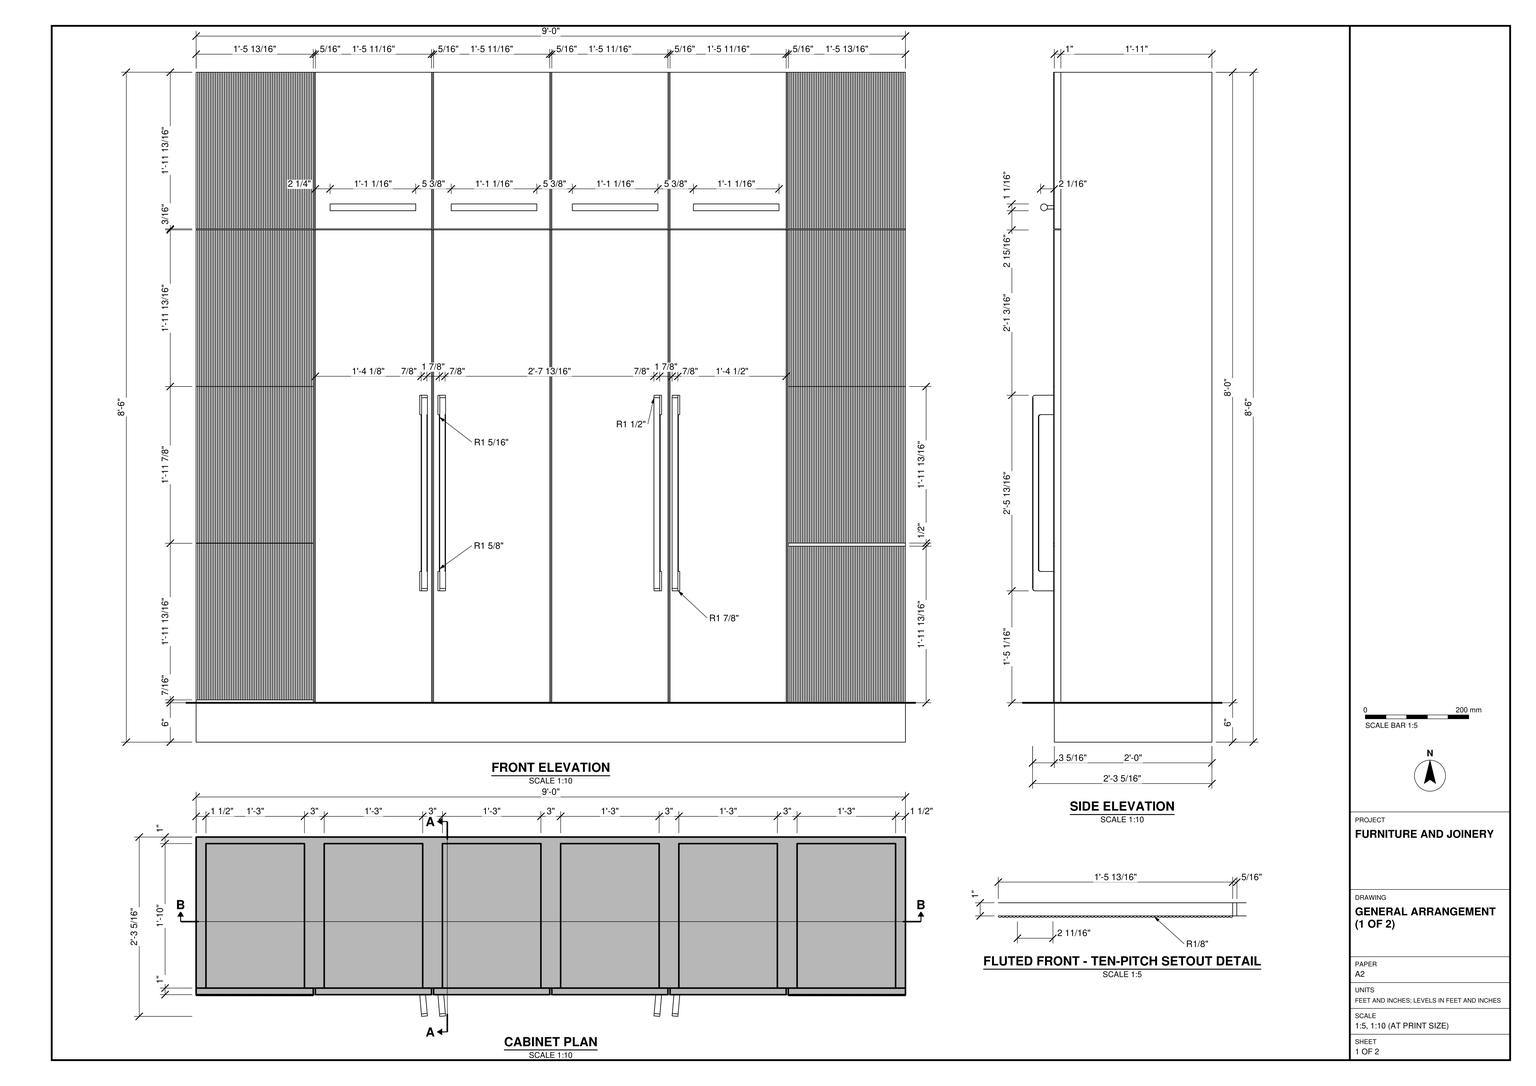
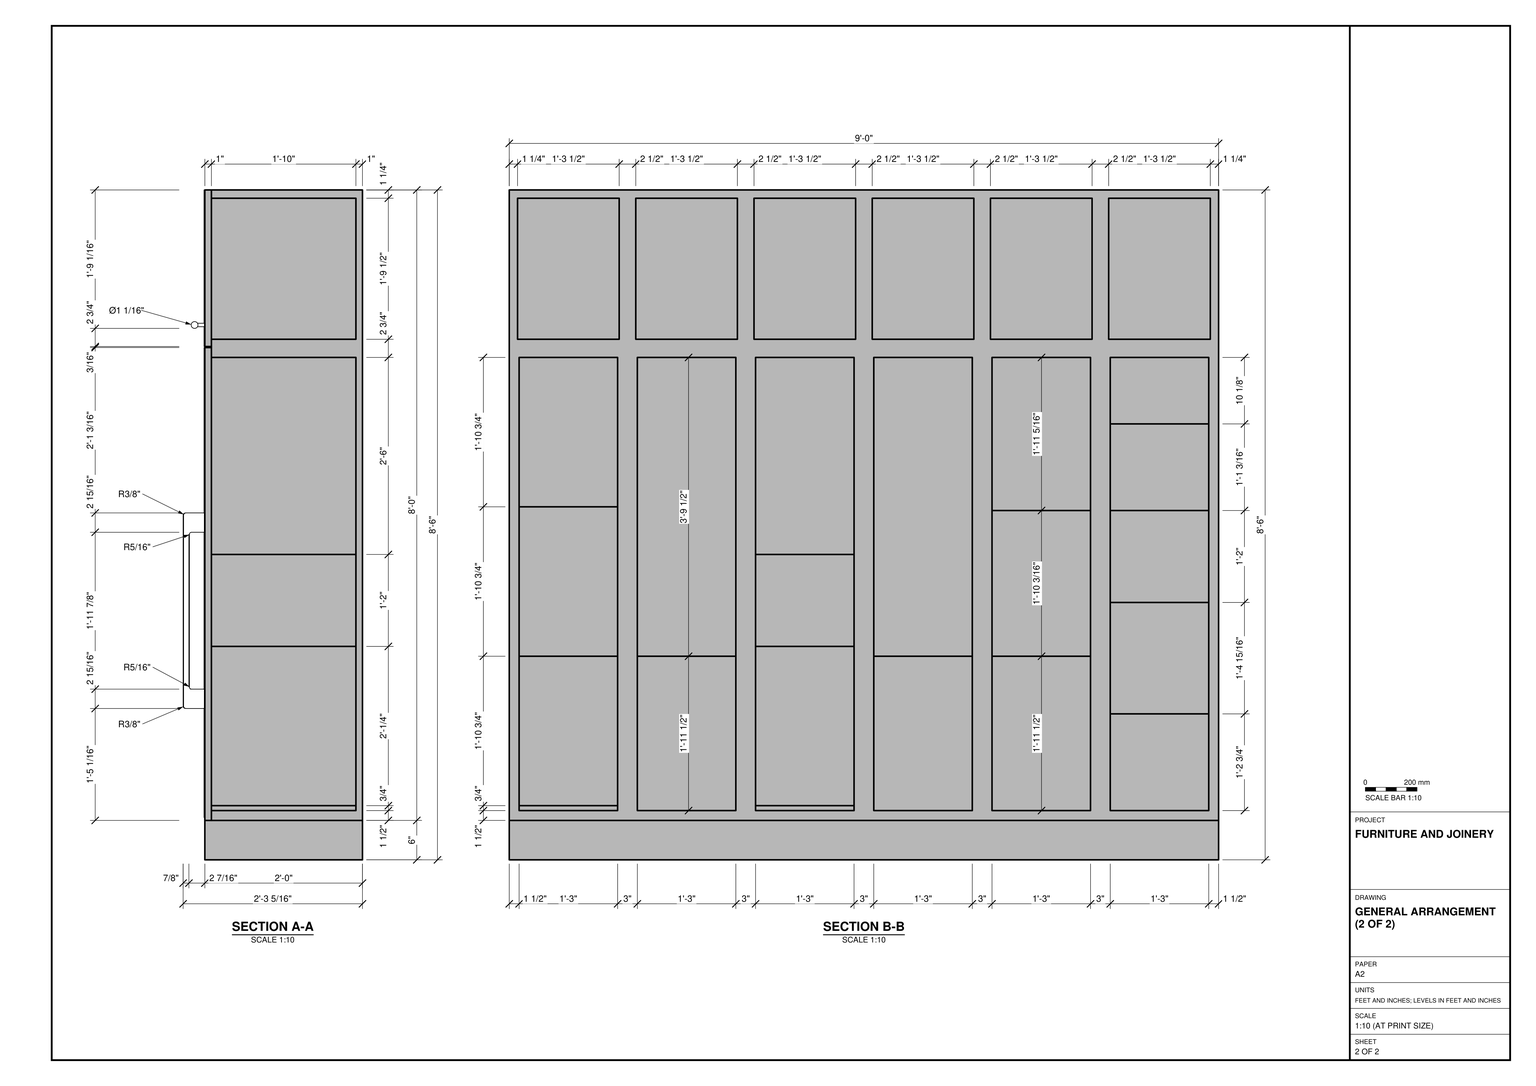
Build the wardrobe in SketchUp from task_files/diagram_01.pdf. Work in feet and inches, with the underside of the plinth at the floor level of ±0'-0". Set the width along the X axis to 9'-0", the overall depth along the Y axis to 2'-3 5/16", and the height to 8'-6". The overall depth includes the projecting pulls; the depth from the back to the closed fronts is 2'-0".

Build the full-width 6" plinth and the cabinet above it. Use the plan and sections to set out the sides, back, top, base, dividers and shelves at the thicknesses shown. Form a row of separate upper compartments and follow section B-B for the shelf heights in each bay below. Do not carry a shelf across a bay that the section shows as open at that height.

Model the fronts closed, keeping the narrow gaps shown in the front elevation. Give the stacked fronts at both ends a vertical fluted profile using the enlarged setout detail. Across the middle, fit short upper doors with horizontal pulls above tall doors with paired vertical pulls. Use the side view to set the pulls clear of the door faces. Keep the cabinet parts, fronts and hardware separately editable as groups or components, and use components for repeated parts. Decor and loose items, if included, may be any suitable library components. Save one SketchUp model as output_files/six_bay_wardrobe_with_fluted_end_fronts.skp.

# SketchUp Ruby script. Lengths in inches.
U = 1.inch
M = Sketchup.active_model
def pt(a) = Geom::Point3d.new(a.map { |v| v * U })
def face(e, loops, mat)
  f = e.add_face(loops[0].map { |a| pt(a) })
  loops[1..].each { |l| e.add_face(l.map { |a| pt(a) }).erase! }
  f.material = f.back_material = mat if mat
  f
end
# faces: each face lists its corners as indices into pts; further lists are holes
def faces(e, pts, list, mat = nil) = list.each { |f| face(e, (f[0].is_a?(Array) ? f : [f]).map { |l| l.map { |i| pts[i] } }, mat) }
# xy, xz, yz: faces in a plane at the given z, y or x. An outline is a flat list of corners, or four numbers for a rectangle; further outlines are holes
def ring(l) = l.size == 4 ? [[l[0], l[1]], [l[2], l[1]], [l[2], l[3]], [l[0], l[3]]] : l.each_slice(2).to_a
def flat(e, list, mat, &to3) = list.each { |f| face(e, (f[0].is_a?(Array) ? f : [f]).map { |l| ring(l).map { |u, v| to3.(u, v) } }, mat) }
def xy(e, z, list, mat = nil) = flat(e, list, mat) { |x, y| [x, y, z] }
def xz(e, y, list, mat = nil) = flat(e, list, mat) { |x, z| [x, y, z] }
def yz(e, x, list, mat = nil) = flat(e, list, mat) { |y, z| [x, y, z] }
def lines(e, pts, list) = list.each { |a, b| e.add_line(pt(pts[a]), pt(pts[b])) }
# prism: a flat outline (further loops are holes) pulled along v
def prism(e, loops, v, mat = nil)
  f = face(e, loops, mat); d = Geom::Vector3d.new(v.map { |x| x * U })
  f.pushpull(f.normal.samedirection?(d) ? d.length : -d.length)
end
def box(e, o, s, mat = nil) = prism(e, [[o, [o[0] + s[0], o[1], o[2]], [o[0] + s[0], o[1] + s[1], o[2]], [o[0], o[1] + s[1], o[2]]]], [0, 0, s[2]], mat)
def at(x, y, z, deg = 0) = Geom::Transformation.translation(pt([x, y, z])) * Geom::Transformation.rotation(ORIGIN, Z_AXIS, deg.degrees)
def axes(o, x, y, z) = Geom::Transformation.new([*x, 0, *y, 0, *z, 0, *pt(o).to_a, 1])
def part(name) = M.definitions.add(name)
# library, detail: a bought-in or finely detailed component or shape, given as its bounding box
def library(name, o, s) = part(name).tap { |d| box(d.entities, o, s) }
def detail(e, o, s) = box(e.add_group.entities, o, s)
def put(e, d, t, mat = nil) = e.add_instance(d, t).tap { |i| i.material = mat if mat }
def group(e, t, mat = nil) = e.add_group.tap { |g| g.transformation = t; g.material = mat if mat }.entities
root = M.entities
M.materials.add("Asian Paints_Archi Concrete Slab Effect_Rocky Terrain").color = [186, 177, 158]
M.materials.add("Asian Paints_Stellato_White Silver").color = [203, 204, 196]
M.materials.add("[0014_DarkSalmon]").color = [233, 150, 122]
M.materials.add("[Color B01]").color = [255, 216, 204]
M.materials.add("[Color C01]").color = [255, 229, 204]
M.materials.add("[Color M09]").color = [0, 0, 0]
M.materials.add("[Granite Dark Gray]").color = [69, 68, 68]
M.materials.add("[Wood Floor Parquet]").color = [142, 87, 38]
c1 = part("tubular wardrobe handle")
g1 = group(c1.entities,at(0,0,0),"[Color B01]")
xy(g1,0,[[0.197,0,0.591,0.984],[0.197,8.858,0.591,9.843]])
xy(g1,0.844,[[0.197,0.984,0.591,8.858]])
xz(g1,0,[[0.197,0,0.591,0,0.591,0.844,0.536,0.814,0.436,0.79,0.333,0.792,0.235,0.821,0.197,0.844],[0.436,0.79,0.536,0.814,0.591,0.844,0.626,0.863,0.7,0.934,0.754,1.022,0.783,1.121,0.784,1.181,0.785,1.223,0.761,1.323,0.712,1.413,0.641,1.488,0.553,1.541,0.454,1.57,0.351,1.573,0.252,1.548,0.161,1.499,0.087,1.428,0.034,1.34,0.005,1.242,0.003,1.181,0.002,1.139,0.027,1.039,0.076,0.949,0.147,0.874,0.197,0.844,0.235,0.821,0.333,0.792]])
xz(g1,0.984,[[0.197,0,0.591,0.844]])
xz(g1,8.858,[[0.197,0,0.591,0.844]])
xz(g1,9.843,[[0.197,0,0.197,0.844,0.235,0.821,0.333,0.792,0.436,0.79,0.536,0.814,0.591,0.844,0.591,0],[0.436,0.79,0.333,0.792,0.235,0.821,0.197,0.844,0.147,0.874,0.076,0.949,0.027,1.039,0.002,1.139,0.005,1.242,0.034,1.34,0.087,1.428,0.161,1.499,0.252,1.548,0.351,1.573,0.454,1.57,0.553,1.541,0.641,1.488,0.712,1.413,0.761,1.323,0.785,1.223,0.783,1.121,0.754,1.022,0.7,0.934,0.626,0.863,0.591,0.844,0.536,0.814]])
yz(g1,0.197,[[0,0,0.984,0.844],[8.858,0,9.843,0.844]])
yz(g1,0.591,[[0,0,0.984,0.844],[8.858,0,9.843,0.844]])
p = [[0.147,9.843,0.874],[0.197,9.843,0.844],[0.197,8.858,0.844],[0.197,0.984,0.844],[0.197,0,0.844],[0.147,0,0.874],
  [0.235,0,0.821],[0.235,9.843,0.821],[0.333,0,0.792],[0.333,9.843,0.792],[0.436,0,0.79],[0.436,9.843,0.79],
  [0.536,0,0.814],[0.536,9.843,0.814],[0.591,0,0.844],[0.591,9.843,0.844],[0.591,8.858,0.844],[0.591,0.984,0.844],
  [0.626,0,0.863],[0.626,9.843,0.863],[0.076,0,0.949],[0.027,0,1.039],[0.027,9.843,1.039],[0.076,9.843,0.949],
  [0.7,0,0.934],[0.7,9.843,0.934],[0.754,0,1.022],[0.754,9.843,1.022],[0.002,0,1.139],[0.002,9.843,1.139],
  [0.783,0,1.121],[0.783,9.843,1.121],[0.003,0,1.181],[0.005,0,1.242],[0.005,9.843,1.242],[0.785,0,1.223],
  [0.784,0,1.181],[0.785,9.843,1.223],[0.034,0,1.34],[0.034,9.843,1.34],[0.761,0,1.323],[0.761,9.843,1.323],
  [0.087,0,1.428],[0.087,9.843,1.428],[0.712,0,1.413],[0.712,9.843,1.413],[0.161,0,1.499],[0.161,9.843,1.499],
  [0.641,0,1.488],[0.641,9.843,1.488],[0.252,0,1.548],[0.252,9.843,1.548],[0.351,0,1.573],[0.351,9.843,1.573],
  [0.454,0,1.57],[0.553,0,1.541],[0.553,9.843,1.541],[0.454,9.843,1.57],[0.787,0,1.181],[0,0,1.181]]
faces(g1,p,[[0,1,2,3,4,5],[6,4,3,2,1,7],[8,6,7,9],[10,8,9,11],[12,10,11,13],[14,12,13,15,16,17],[18,14,17,16,15,19],[20,21,22,23],
  [5,20,23,0],[24,18,19,25],[26,24,25,27],[21,28,29,22],[30,26,27,31],[28,32,33,34,29],[35,36,30,31,37],[33,38,39,34],
  [40,35,37,41],[38,42,43,39],[44,40,41,45],[42,46,47,43],[48,44,45,49],[46,50,51,47],[50,52,53,51],[54,55,56,57],
  [55,48,49,56],[52,54,57,53]])
lines(g1,p,[[58,36],[59,32]])
c2 = part("Modern+Drawer+Handle+10+inch+01")
g2 = group(c2.entities,at(0,0,0),"[Color C01]")
yz(g2,0,[[-1,-0.09,-1.03,0.21,-1.01,0.21,-0.99,-0.09],[-0.99,-0.09,-1.01,0.21,-1,0.21,-0.97,-0.08],[-0.97,-0.08,-1,0.21,-0.03,0.3,0,0]])
yz(g2,1,[[-0.72,-0.0625,-0.71,-0.0625,-0.73,0.24,-0.75,0.24],[-0.71,-0.0625,-0.6875,-0.06,-0.72,0.24,-0.73,0.24],[-0.6875,-0.06,-0.67,-0.06,-0.7,0.24,-0.72,0.24],[-0.67,-0.06,0,0,-0.03,0.3,-0.7,0.24]])
yz(g2,9.1,[[-0.72,-0.0625,-0.75,0.24,-0.73,0.24,-0.71,-0.0625],[-0.71,-0.0625,-0.73,0.24,-0.72,0.24,-0.6875,-0.06],[-0.6875,-0.06,-0.72,0.24,-0.7,0.24,-0.67,-0.06],[-0.67,-0.06,-0.7,0.24,-0.03,0.3,0,0]])
yz(g2,10.1,[[-1,-0.09,-0.99,-0.09,-1.01,0.21,-1.03,0.21],[-0.99,-0.09,-0.97,-0.08,-1,0.21,-1.01,0.21],[-0.97,-0.08,0,0,-0.03,0.3,-1,0.21]])
p = [[0.04,-1.06,-0.09],[0.05,-1.07,-0.09],[0.05,-1.1,0.21],[0.04,-1.09,0.21],[0.02,-1.03,-0.09],[0.03,-1.05,-0.09],
  [0.03,-1.07,0.21],[0.02,-1.06,0.21],[0.0625,-1.08,-0.09],[0.0625,-1.11,0.2],[9.97,-1.1,-0.1],[0.125,-1.1,-0.1],
  [0.11,-1.09,-0.1],[0.09,-1.09,-0.1],[0.08,-1.09,-0.1],[0.01,-1.02,-0.09],[0,-1,-0.09],[0,-0.99,-0.09],
  [0,-0.97,-0.08],[0,0,0],[1,0,0],[1,-0.67,-0.06],[1,-0.6875,-0.06],[1,-0.71,-0.0625],
  [1,-0.72,-0.0625],[1.01,-0.74,-0.06],[1.02,-0.75,-0.07],[1.03,-0.77,-0.07],[1.04,-0.78,-0.07],[1.06,-0.79,-0.07],
  [1.07,-0.79,-0.07],[1.09,-0.8,-0.07],[1.11,-0.8,-0.07],[1.125,-0.8,-0.07],[8.97,-0.8,-0.07],[8.99,-0.8,-0.07],
  [9.01,-0.8,-0.07],[9.03,-0.79,-0.07],[9.04,-0.79,-0.07],[9.06,-0.78,-0.07],[9.07,-0.77,-0.07],[9.08,-0.75,-0.07],
  [9.09,-0.74,-0.06],[9.1,-0.72,-0.0625],[9.1,-0.71,-0.0625],[9.1,-0.6875,-0.06],[9.1,-0.67,-0.06],[9.1,0,0],
  [10.1,0,0],[10.1,-0.97,-0.08],[10.1,-0.99,-0.09],[10.1,-1,-0.09],[10.09,-1.02,-0.09],[10.08,-1.03,-0.09],
  [10.07,-1.05,-0.09],[10.0625,-1.06,-0.09],[10.05,-1.07,-0.09],[10.04,-1.08,-0.09],[10.02,-1.09,-0.1],[10.01,-1.09,-0.1],
  [9.99,-1.09,-0.1],[0.01,-1.05,0.21],[9.97,-1.12,0.2],[0.125,-1.12,0.2],[0.11,-1.12,0.2],[0.09,-1.12,0.2],
  [0.08,-1.11,0.2],[10.01,-1.12,0.2],[9.99,-1.12,0.2],[10.04,-1.11,0.2],[10.02,-1.11,0.2],[10.05,-1.1,0.21],
  [10.08,-1.06,0.21],[10.07,-1.07,0.21],[10.0625,-1.09,0.21],[10.09,-1.05,0.21],[0,-1.03,0.21],[10.1,-1.03,0.21],
  [1.01,-0.76,0.23],[1.02,-0.78,0.23],[1.03,-0.79,0.23],[1.04,-0.8,0.23],[1.06,-0.8125,0.23],[1,-0.75,0.24],
  [1.07,-0.82,0.23],[1.09,-0.82,0.23],[1.11,-0.82,0.23],[1.125,-0.82,0.23],[8.97,-0.82,0.23],[8.99,-0.82,0.23],
  [9.01,-0.82,0.23],[9.03,-0.82,0.23],[9.04,-0.8125,0.23],[9.06,-0.8,0.23],[9.07,-0.79,0.23],[9.08,-0.78,0.23],
  [9.09,-0.76,0.23],[9.1,-0.75,0.24],[0,-0.03,0.3],[1,-0.03,0.3],[9.1,-0.03,0.3],[10.1,-0.03,0.3],
  [9.1,-0.7,0.24],[9.1,-0.72,0.24],[9.1,-0.73,0.24],[1,-0.73,0.24],[1,-0.72,0.24],[1,-0.7,0.24],
  [0,-1,0.21],[0,-1.01,0.21],[10.1,-1.01,0.21],[10.1,-1,0.21]]
faces(g2,p,[[0,1,2,3],[4,5,6,7],[1,8,9,2],[5,0,3,6],[10,11,12,13,14,8,1,0,5,4,15,16,17,18,19,20,21,22,23,24,25,26,27,28,29,30,31,32,33,34,35,36,37,38,39,40,41,42,43,44,45,46,47,48,49,50,51,52,53,54,55,56,57,58,59,60],[15,4,7,61],[13,12,64,65],[8,14,66,9],
  [12,11,63,64],[14,13,65,66],[60,59,67,68],[58,57,69,70],[57,56,71,69],[59,58,70,67],[10,60,68,62],[54,53,72,73],
  [56,55,74,71],[55,54,73,74],[53,52,75,72],[16,15,61,76],[52,51,77,75],[26,25,78,79],[28,27,80,81],[29,28,81,82],
  [25,24,83,78],[27,26,79,80],[31,30,84,85],[33,32,86,87],[32,31,85,86],[34,33,87,88],[30,29,82,84],[35,34,88,89],
  [37,36,90,91],[36,35,89,90],[39,38,92,93],[38,37,91,92],[41,40,94,95],[40,39,93,94],[43,42,96,97],[42,41,95,96],
  [98,99,20,19],[47,100,101,48],[101,100,102,103,104,97,96,95,94,93,92,91,90,89,88,87,86,85,84,82,81,80,79,78,83,105,106,107,99,98,108,109,76,61,7,6,3,2,9,66,65,64,63,62,68,67,70,69,71,74,73,72,75,77,110,111]])
faces(g2,p,[[10,62,63,11]],"[Color C01]")
c3 = part("Fluting strip")
xy(c3.entities,-23.84,[[0.09,0,0.0625,0.02,0.04,0.04,0.02,0.0625,0,0.09,0,0.125,0.25,0.125,0.25,0.09,0.23,0.0625,0.21,0.04,0.1875,0.02,0.16,0]])
xy(c3.entities,0,[[0.09,0,0.16,0,0.1875,0.02,0.21,0.04,0.23,0.0625,0.25,0.09,0.25,0.125,0,0.125,0,0.09,0.02,0.0625,0.04,0.04,0.0625,0.02]])
xz(c3.entities,0,[[0.09,-23.84,0.125,0],[0.125,-23.84,0.16,0]],"[0014_DarkSalmon]")
xz(c3.entities,0.125,[[0,-23.84,0.25,0]])
yz(c3.entities,0,[[0.09,-23.84,0.125,0]],"[0014_DarkSalmon]")
yz(c3.entities,0.25,[[0.09,-23.84,0.125,0]],"[0014_DarkSalmon]")
p = [[0.04,0.04,0],[0.02,0.0625,0],[0.02,0.0625,-23.84],[0.04,0.04,-23.84],[0.0625,0.02,0],[0.0625,0.02,-23.84],
  [0.09,0,0],[0.09,0,-23.84],[0.1875,0.02,0],[0.16,0,0],[0.16,0,-23.84],[0.1875,0.02,-23.84],
  [0.21,0.04,0],[0.21,0.04,-23.84],[0.23,0.0625,0],[0.23,0.0625,-23.84],[0,0.09,0],[0,0.09,-23.84],
  [0.25,0.09,0],[0.25,0.09,-23.84]]
faces(c3.entities,p,[[0,1,2,3],[4,0,3,5],[6,4,5,7],[8,9,10,11],[12,8,11,13],[14,12,13,15],[1,16,17,2],[18,14,15,19]],"[0014_DarkSalmon]")
c4 = part("Fluted front panel")
put(c4.entities,c3,at(11.91,0,23.84))
put(c4.entities,c3,at(12.18,0,23.84))
put(c4.entities,c3,at(7.85,0,23.84))
put(c4.entities,c3,at(8.39,0,23.84))
put(c4.entities,c3,at(12.72,0,23.84))
put(c4.entities,c3,at(4.87,0,23.84))
put(c4.entities,c3,at(6.77,0,23.84))
put(c4.entities,c3,at(3.79,0,23.84))
put(c4.entities,c3,at(1.89,0,23.84))
put(c4.entities,c3,at(7.31,0,23.84))
put(c4.entities,c3,at(2.4375,0,23.84))
put(c4.entities,c3,at(3.25,0,23.84))
put(c4.entities,c3,at(6.5,0,23.84))
put(c4.entities,c3,at(0.27,0,23.84))
put(c4.entities,c3,at(0.54,0,23.84))
put(c4.entities,c3,at(3.52,0,23.84))
put(c4.entities,c3,at(10.28,0,23.84))
put(c4.entities,c3,at(9.74,0,23.84))
put(c4.entities,c3,at(8.66,0,23.84))
put(c4.entities,c3,at(10.83,0,23.84))
put(c4.entities,c3,at(10.01,0,23.84))
put(c4.entities,c3,at(0,0,23.84))
put(c4.entities,c3,at(14.34,0,23.84))
put(c4.entities,c3,at(7.58,0,23.84))
put(c4.entities,c3,at(8.93,0,23.84))
put(c4.entities,c3,at(11.64,0,23.84))
put(c4.entities,c3,at(17.05,0,23.84))
put(c4.entities,c3,at(16.51,0,23.84))
put(c4.entities,c3,at(17.59,0,23.84))
put(c4.entities,c3,at(16.78,0,23.84))
put(c4.entities,c3,at(17.32,0,23.84))
put(c4.entities,c3,at(15.7,0,23.84))
put(c4.entities,c3,at(14.62,0,23.84))
put(c4.entities,c3,at(13.26,0,23.84))
put(c4.entities,c3,at(14.07,0,23.84))
put(c4.entities,c3,at(8.12,0,23.84))
put(c4.entities,c3,at(10.56,0,23.84))
put(c4.entities,c3,at(11.1,0,23.84))
put(c4.entities,c3,at(9.2,0,23.84))
put(c4.entities,c3,at(12.99,0,23.84))
put(c4.entities,c3,at(5.95,0,23.84))
put(c4.entities,c3,at(5.68,0,23.84))
put(c4.entities,c3,at(1.08,0,23.84))
put(c4.entities,c3,at(5.41,0,23.84))
put(c4.entities,c3,at(4.06,0,23.84))
put(c4.entities,c3,at(1.35,0,23.84))
put(c4.entities,c3,at(1.625,0,23.84))
put(c4.entities,c3,at(2.71,0,23.84))
put(c4.entities,c3,at(4.6,0,23.84))
put(c4.entities,c3,at(2.17,0,23.84))
put(c4.entities,c3,at(0.8125,0,23.84))
put(c4.entities,c3,at(4.33,0,23.84))
put(c4.entities,c3,at(5.14,0,23.84))
put(c4.entities,c3,at(9.47,0,23.84))
put(c4.entities,c3,at(13.8,0,23.84))
put(c4.entities,c3,at(11.37,0,23.84))
put(c4.entities,c3,at(13.53,0,23.84))
put(c4.entities,c3,at(12.45,0,23.84))
put(c4.entities,c3,at(15.97,0,23.84))
put(c4.entities,c3,at(16.24,0,23.84))
put(c4.entities,c3,at(14.89,0,23.84))
put(c4.entities,c3,at(15.16,0,23.84))
put(c4.entities,c3,at(15.43,0,23.84))
put(c4.entities,c3,at(7.04,0,23.84))
put(c4.entities,c3,at(2.98,0,23.84))
put(c4.entities,c3,at(6.23,0,23.84))
c5 = part("Group\#7")
xy(c5.entities,0.75,[[0,0,15,22]])
xz(c5.entities,0,[[0,0,15,0.75]])
p = [[18,4.31,23.375],[18.31,4.31,23.375]]
lines(root,p,[[0,1]])
put(root,c1,axes([33.4375,3.31,80.92],[0,0,1.32422],[-1.32422,0,0],[0,-1.32422,0]))
put(root,c2,axes([34.93,3.31,23.04],[0,0,2.94868],[0,2.94868,0],[-2.94868,0,0]))
put(root,c2,axes([37.7,3.31,23.04],[0,0,2.94868],[0,2.94868,0],[-2.94868,0,0]))
put(root,c2,axes([72.75,3.31,23.04],[0,0,2.94868],[0,2.94868,0],[2.94868,0,0]))
put(root,c2,axes([69.99,3.31,23.04],[0,0,2.94868],[0,2.94868,0],[2.94868,0,0]))
put(root,c1,axes([51.875,3.31,80.92],[0,0,1.32422],[-1.32422,0,0],[0,-1.32422,0]))
put(root,c1,axes([70.3125,3.31,80.92],[0,0,1.32422],[-1.32422,0,0],[0,-1.32422,0]))
put(root,c1,axes([88.75,3.31,80.92],[0,0,1.32422],[-1.32422,0,0],[0,-1.32422,0]))
g3 = group(root,at(0,3.31,0))
xy(g3,0,[[0,0,108,24]])
xy(g3,6,[[0,0,108,24]],"[Granite Dark Gray]")
xz(g3,0,[[0,0,108,6]],"[Granite Dark Gray]")
xz(g3,24,[[0,0,108,6]],"[Granite Dark Gray]")
yz(g3,0,[[0,0,24,6]],"[Granite Dark Gray]")
yz(g3,108,[[0,0,24,6]],"[Granite Dark Gray]")
g4 = group(root,at(0,3.31,6))
xy(g4,0,[[0,0,17.84,1],[18.16,0,35.84,1],[36.16,0,53.84,1],[54.16,0,71.84,1],[72.16,0,89.84,1],
  [90.16,0,108,1]])
xy(g4,72,[[0,0,17.84,1],[18.16,0,35.84,1],[36.16,0,53.84,1],[54.16,0,71.84,1],[72.16,0,89.84,1],
  [90.16,0,108,1]])
xy(g4,72.16,[[0,0,17.84,1],[18.16,0,35.84,1],[36.16,0,53.84,1],[54.16,0,71.84,1],[72.16,0,89.84,1],
  [90.16,0,107.84,1],[107.84,0,108,1]])
xy(g4,96,[[0,0,17.84,1],[18.16,0,35.84,1],[36.16,0,53.84,1],[54.16,0,71.84,1],[72.16,0,89.84,1],
  [90.16,0,108,1]])
xz(g4,0,[[0,0,17.84,72],[90.16,0,108,72],[0,72.16,17.84,96],[90.16,72.16,108,96]])
xz(g4,0,[[18.16,0,35.84,72],[36.16,0,53.84,72],[54.16,0,71.84,72],[72.16,0,89.84,72],[18.16,72.16,35.84,96],
  [36.16,72.16,53.84,96],[54.16,72.16,71.84,96],[72.16,72.16,89.84,96]],"Asian Paints_Stellato_White Silver")
xz(g4,1,[[0,0,17.84,72],[17.84,0,18.16,72],[18.16,0,35.84,72],[35.84,0,36.16,72],[36.16,0,53.84,72],
  [53.84,0,54.16,72],[54.16,0,71.84,72],[71.84,0,72.16,72],[72.16,0,89.84,72],[90.16,0,108,72],
  [0,72,17.84,72.16],[18.16,72,35.84,72.16],[36.16,72,53.84,72.16],[54.16,72,71.84,72.16],[72.16,72,89.84,72.16],
  [90.16,72,108,72.16],[0,72.16,17.84,96],[18.16,72.16,35.84,96],[36.16,72.16,53.84,96],[54.16,72.16,71.84,96],
  [72.16,72.16,89.84,96],[90.16,72.16,108,96]])
yz(g4,0,[[0,0,1,72],[0,72.16,1,96]])
yz(g4,17.84,[[0,0,1,72],[0,72.16,1,96]])
yz(g4,18.16,[[0,0,1,72],[0,72.16,1,96]])
yz(g4,35.84,[[0,0,1,72],[0,72.16,1,96]])
yz(g4,36.16,[[0,0,1,72],[0,72.16,1,96]])
yz(g4,53.84,[[0,0,1,72],[0,72.16,1,96]])
yz(g4,54.16,[[0,0,1,72],[0,72.16,1,96]])
yz(g4,71.84,[[0,0,1,72],[0,72.16,1,96]])
yz(g4,72.16,[[0,0,1,72],[0,72.16,1,96]])
yz(g4,89.84,[[0,0,1,72],[0,72.16,1,96]])
yz(g4,90.16,[[0,0,1,72],[0,72.16,1,96]])
yz(g4,108,[[0,0,1,72],[0,72.16,1,96]])
p = [[89.84,1,0],[90.16,1,0]]
lines(g4,p,[[0,1]])
g5 = group(root,at(0,3.18,6.44))
put(g5,c3,at(0,0,95.56))
put(g5,c4,at(0,0,47.72))
put(g5,c4,at(0,0,0))
put(g5,c4,at(0,0,23.875))
put(g5,c3,at(9.74,0,95.56))
put(g5,c3,at(10.01,0,95.56))
put(g5,c3,at(10.28,0,95.56))
put(g5,c3,at(8.66,0,95.56))
put(g5,c3,at(11.64,0,95.56))
put(g5,c3,at(14.34,0,95.56))
put(g5,c3,at(7.58,0,95.56))
put(g5,c3,at(8.93,0,95.56))
put(g5,c3,at(10.83,0,95.56))
put(g5,c3,at(9.2,0,95.56))
put(g5,c3,at(12.99,0,95.56))
put(g5,c3,at(10.56,0,95.56))
put(g5,c3,at(14.62,0,95.56))
put(g5,c3,at(14.07,0,95.56))
put(g5,c3,at(8.12,0,95.56))
put(g5,c3,at(11.1,0,95.56))
put(g5,c3,at(7.85,0,95.56))
put(g5,c3,at(11.91,0,95.56))
put(g5,c3,at(12.18,0,95.56))
put(g5,c3,at(8.39,0,95.56))
put(g5,c3,at(12.72,0,95.56))
put(g5,c3,at(13.26,0,95.56))
put(g5,c3,at(9.47,0,95.56))
put(g5,c3,at(11.37,0,95.56))
put(g5,c3,at(13.8,0,95.56))
put(g5,c3,at(13.53,0,95.56))
put(g5,c3,at(12.45,0,95.56))
put(g5,c3,at(7.04,0,95.56))
put(g5,c3,at(6.23,0,95.56))
put(g5,c3,at(2.98,0,95.56))
put(g5,c3,at(7.31,0,95.56))
put(g5,c3,at(1.89,0,95.56))
put(g5,c3,at(4.87,0,95.56))
put(g5,c3,at(0.27,0,95.56))
put(g5,c3,at(3.25,0,95.56))
put(g5,c3,at(3.52,0,95.56))
put(g5,c3,at(6.77,0,95.56))
put(g5,c3,at(3.79,0,95.56))
put(g5,c3,at(6.5,0,95.56))
put(g5,c3,at(2.4375,0,95.56))
put(g5,c3,at(0.54,0,95.56))
put(g5,c3,at(4.06,0,95.56))
put(g5,c3,at(2.71,0,95.56))
put(g5,c3,at(0.8125,0,95.56))
put(g5,c3,at(1.625,0,95.56))
put(g5,c3,at(2.17,0,95.56))
put(g5,c3,at(4.33,0,95.56))
put(g5,c3,at(5.41,0,95.56))
put(g5,c3,at(4.6,0,95.56))
put(g5,c3,at(1.35,0,95.56))
put(g5,c3,at(5.14,0,95.56))
put(g5,c3,at(5.95,0,95.56))
put(g5,c3,at(5.68,0,95.56))
put(g5,c3,at(1.08,0,95.56))
put(g5,c3,at(15.16,0,95.56))
put(g5,c3,at(15.43,0,95.56))
put(g5,c3,at(15.97,0,95.56))
put(g5,c3,at(16.24,0,95.56))
put(g5,c3,at(14.89,0,95.56))
put(g5,c3,at(16.51,0,95.56))
put(g5,c3,at(15.7,0,95.56))
put(g5,c3,at(17.05,0,95.56))
put(g5,c3,at(16.78,0,95.56))
put(g5,c3,at(17.59,0,95.56))
put(g5,c3,at(17.32,0,95.56))
g6 = group(root,at(90.16,3.18,6))
put(g6,c3,at(11.64,0,23.84))
put(g6,c3,at(10.01,0,23.84))
put(g6,c3,at(14.89,0,23.84))
put(g6,c3,at(16.51,0,23.84))
put(g6,c3,at(8.66,0,23.84))
put(g6,c3,at(15.43,0,23.84))
put(g6,c3,at(5.68,0,23.84))
put(g6,c3,at(0.54,0,23.84))
put(g6,c3,at(16.24,0,23.84))
put(g6,c3,at(17.59,0,23.84))
put(g6,c3,at(8.93,0,23.84))
put(g6,c3,at(8.12,0,23.84))
put(g6,c3,at(1.625,0,23.84))
put(g6,c3,at(15.7,0,23.84))
put(g6,c3,at(5.41,0,23.84))
put(g6,c3,at(0.8125,0,23.84))
put(g6,c3,at(5.14,0,23.84))
put(g6,c3,at(1.08,0,23.84))
put(g6,c3,at(9.47,0,23.84))
put(g6,c3,at(0,0,23.84))
put(g6,c3,at(10.83,0,23.84))
put(g6,c3,at(1.35,0,23.84))
put(g6,c3,at(16.78,0,23.84))
put(g6,c3,at(10.28,0,23.84))
put(g6,c3,at(14.62,0,23.84))
put(g6,c3,at(5.95,0,23.84))
put(g6,c3,at(17.05,0,23.84))
put(g6,c3,at(17.32,0,23.84))
put(g6,c3,at(15.16,0,23.84))
put(g6,c3,at(15.97,0,23.84))
put(g6,c3,at(4.6,0,23.84))
put(g6,c3,at(9.2,0,23.84))
put(g6,c3,at(12.99,0,23.84))
put(g6,c3,at(2.71,0,72))
put(g6,c3,at(2.4375,0,72))
put(g6,c3,at(4.06,0,72))
put(g6,c3,at(0.54,0,48.16))
put(g6,c3,at(0.27,0,23.84))
put(g6,c3,at(14.89,0,48.16))
put(g6,c3,at(2.17,0,23.84))
put(g6,c3,at(16.24,0,48.16))
put(g6,c3,at(8.93,0,48.16))
put(g6,c3,at(15.7,0,48.16))
put(g6,c3,at(4.06,0,23.84))
put(g6,c3,at(8.66,0,48.16))
put(g6,c3,at(15.43,0,48.16))
put(g6,c3,at(5.41,0,48.16))
put(g6,c3,at(0.8125,0,48.16))
put(g6,c3,at(5.14,0,48.16))
put(g6,c3,at(1.08,0,48.16))
put(g6,c3,at(9.47,0,48.16))
put(g6,c3,at(0,0,48.16))
put(g6,c3,at(2.4375,0,48.16))
put(g6,c3,at(1.625,0,48.16))
put(g6,c3,at(17.59,0,48.16))
put(g6,c3,at(2.71,0,23.84))
put(g6,c3,at(6.5,0,23.84))
put(g6,c3,at(3.25,0,23.84))
put(g6,c3,at(8.12,0,48.16))
put(g6,c3,at(11.64,0,48.16))
put(g6,c3,at(5.68,0,48.16))
put(g6,c3,at(3.79,0,23.84))
put(g6,c3,at(6.77,0,23.84))
put(g6,c3,at(8.39,0,23.84))
put(g6,c3,at(16.51,0,48.16))
put(g6,c3,at(10.01,0,48.16))
put(g6,c3,at(2.4375,0,23.84))
put(g6,c3,at(2.17,0,96))
put(g6,c3,at(10.56,0,48.16))
put(g6,c3,at(13.8,0,48.16))
put(g6,c3,at(6.23,0,48.16))
put(g6,c3,at(12.45,0,48.16))
put(g6,c3,at(12.72,0,48.16))
put(g6,c3,at(14.34,0,48.16))
put(g6,c3,at(7.04,0,48.16))
put(g6,c3,at(11.37,0,48.16))
put(g6,c3,at(12.18,0,48.16))
put(g6,c3,at(4.33,0,48.16))
put(g6,c3,at(4.87,0,48.16))
put(g6,c3,at(7.85,0,48.16))
put(g6,c3,at(9.74,0,48.16))
put(g6,c3,at(2.98,0,48.16))
put(g6,c3,at(13.26,0,48.16))
put(g6,c3,at(11.91,0,48.16))
put(g6,c3,at(13.53,0,48.16))
put(g6,c3,at(7.58,0,48.16))
put(g6,c3,at(1.89,0,48.16))
put(g6,c3,at(11.1,0,48.16))
put(g6,c3,at(14.07,0,48.16))
put(g6,c3,at(7.31,0,48.16))
put(g6,c3,at(3.52,0,48.16))
put(g6,c3,at(2.71,0,48.16))
put(g6,c3,at(6.5,0,48.16))
put(g6,c3,at(3.25,0,48.16))
put(g6,c3,at(3.79,0,48.16))
put(g6,c3,at(6.5,0,72))
put(g6,c3,at(3.79,0,72))
put(g6,c3,at(3.25,0,72))
put(g6,c3,at(6.77,0,72))
put(g6,c3,at(0.27,0,72))
put(g6,c3,at(10.28,0,48.16))
put(g6,c3,at(5.95,0,48.16))
put(g6,c3,at(14.34,0,23.84))
put(g6,c3,at(4.33,0,23.84))
put(g6,c3,at(7.04,0,23.84))
put(g6,c3,at(12.18,0,23.84))
put(g6,c3,at(14.07,0,23.84))
put(g6,c3,at(7.31,0,23.84))
put(g6,c3,at(15.97,0,48.16))
put(g6,c3,at(2.98,0,23.84))
put(g6,c3,at(17.05,0,48.16))
put(g6,c3,at(1.35,0,48.16))
put(g6,c3,at(6.23,0,23.84))
put(g6,c3,at(3.52,0,23.84))
put(g6,c3,at(10.56,0,23.84))
put(g6,c3,at(13.26,0,23.84))
put(g6,c3,at(4.87,0,23.84))
put(g6,c3,at(10.83,0,48.16))
put(g6,c3,at(14.62,0,48.16))
put(g6,c3,at(9.74,0,23.84))
put(g6,c3,at(17.32,0,48.16))
put(g6,c3,at(15.16,0,48.16))
put(g6,c3,at(7.85,0,23.84))
put(g6,c3,at(12.45,0,23.84))
put(g6,c3,at(11.37,0,23.84))
put(g6,c3,at(16.78,0,48.16))
put(g6,c3,at(13.8,0,23.84))
put(g6,c3,at(7.58,0,23.84))
put(g6,c3,at(11.1,0,23.84))
put(g6,c3,at(1.89,0,23.84))
put(g6,c3,at(11.91,0,23.84))
put(g6,c3,at(12.72,0,23.84))
put(g6,c3,at(13.53,0,23.84))
put(g6,c3,at(2.17,0,72))
put(g6,c3,at(0.8125,0,72))
put(g6,c3,at(0.54,0,72))
put(g6,c3,at(1.625,0,72))
put(g6,c3,at(0.54,0,96))
put(g6,c3,at(0.8125,0,96))
put(g6,c3,at(1.625,0,96))
put(g6,c3,at(2.4375,0,96))
put(g6,c3,at(4.06,0,96))
put(g6,c3,at(2.71,0,96))
put(g6,c3,at(15.43,0,96))
put(g6,c3,at(1.35,0,96))
put(g6,c3,at(5.95,0,96))
put(g6,c3,at(5.68,0,96))
put(g6,c3,at(1.08,0,96))
put(g6,c3,at(14.89,0,96))
put(g6,c3,at(4.6,0,96))
put(g6,c3,at(16.51,0,96))
put(g6,c3,at(15.16,0,96))
put(g6,c3,at(15.7,0,96))
put(g6,c3,at(15.97,0,96))
put(g6,c3,at(17.05,0,96))
put(g6,c3,at(16.78,0,96))
put(g6,c3,at(5.41,0,96))
put(g6,c3,at(17.59,0,96))
put(g6,c3,at(17.32,0,96))
put(g6,c3,at(5.14,0,96))
put(g6,c3,at(16.24,0,96))
put(g6,c3,at(9.2,0,48.16))
put(g6,c3,at(4.6,0,48.16))
put(g6,c3,at(12.99,0,48.16))
put(g6,c3,at(0.27,0,48.16))
put(g6,c3,at(2.17,0,48.16))
put(g6,c3,at(4.06,0,48.16))
put(g6,c3,at(9.47,0,96))
put(g6,c3,at(13.26,0,96))
put(g6,c3,at(12.72,0,96))
put(g6,c3,at(6.23,0,96))
put(g6,c3,at(13.8,0,96))
put(g6,c3,at(2.98,0,96))
put(g6,c3,at(7.31,0,96))
put(g6,c3,at(4.87,0,96))
put(g6,c3,at(13.53,0,96))
put(g6,c3,at(11.37,0,96))
put(g6,c3,at(7.04,0,96))
put(g6,c3,at(12.45,0,96))
put(g6,c3,at(1.89,0,96))
put(g6,c3,at(17.05,0,72))
put(g6,c3,at(5.41,0,72))
put(g6,c3,at(15.7,0,72))
put(g6,c3,at(17.32,0,72))
put(g6,c3,at(5.14,0,72))
put(g6,c3,at(16.78,0,72))
put(g6,c3,at(1.08,0,72))
put(g6,c3,at(15.16,0,72))
put(g6,c3,at(5.68,0,72))
put(g6,c3,at(14.89,0,72))
put(g6,c3,at(16.51,0,72))
put(g6,c3,at(15.97,0,72))
put(g6,c3,at(17.59,0,72))
put(g6,c3,at(16.24,0,72))
put(g6,c3,at(4.6,0,72))
put(g6,c3,at(9.47,0,72))
put(g6,c3,at(8.39,0,48.16))
put(g6,c3,at(9.2,0,72))
put(g6,c3,at(0,0,72))
put(g6,c3,at(8.93,0,72))
put(g6,c3,at(11.64,0,72))
put(g6,c3,at(12.99,0,72))
put(g6,c3,at(8.66,0,72))
put(g6,c3,at(6.77,0,48.16))
put(g6,c3,at(10.28,0,72))
put(g6,c3,at(10.01,0,72))
put(g6,c3,at(3.52,0,96))
put(g6,c3,at(6.77,0,96))
put(g6,c3,at(3.79,0,96))
put(g6,c3,at(6.5,0,96))
put(g6,c3,at(0.27,0,96))
put(g6,c3,at(3.25,0,96))
put(g6,c3,at(10.83,0,96))
put(g6,c3,at(14.62,0,96))
put(g6,c3,at(8.12,0,96))
put(g6,c3,at(9.74,0,96))
put(g6,c3,at(14.34,0,96))
put(g6,c3,at(11.1,0,96))
put(g6,c3,at(7.85,0,96))
put(g6,c3,at(12.18,0,96))
put(g6,c3,at(14.07,0,96))
put(g6,c3,at(8.39,0,96))
put(g6,c3,at(10.56,0,96))
put(g6,c3,at(7.58,0,96))
put(g6,c3,at(11.91,0,96))
put(g6,c3,at(4.33,0,96))
put(g6,c3,at(9.2,0,96))
put(g6,c3,at(12.99,0,96))
put(g6,c3,at(8.66,0,96))
put(g6,c3,at(10.01,0,96))
put(g6,c3,at(0,0,96))
put(g6,c3,at(8.93,0,96))
put(g6,c3,at(10.28,0,96))
put(g6,c3,at(11.64,0,96))
put(g6,c3,at(10.83,0,72))
put(g6,c3,at(14.62,0,72))
put(g6,c3,at(8.12,0,72))
put(g6,c3,at(1.35,0,72))
put(g6,c3,at(5.95,0,72))
put(g6,c3,at(15.43,0,72))
put(g6,c3,at(8.39,0,72))
put(g6,c3,at(14.34,0,72))
put(g6,c3,at(7.58,0,72))
put(g6,c3,at(11.91,0,72))
put(g6,c3,at(7.85,0,72))
put(g6,c3,at(10.56,0,72))
put(g6,c3,at(12.18,0,72))
put(g6,c3,at(14.07,0,72))
put(g6,c3,at(4.33,0,72))
put(g6,c3,at(9.74,0,72))
put(g6,c3,at(11.1,0,72))
put(g6,c3,at(1.89,0,72))
put(g6,c3,at(6.23,0,72))
put(g6,c3,at(2.98,0,72))
put(g6,c3,at(11.37,0,72))
put(g6,c3,at(7.31,0,72))
put(g6,c3,at(3.52,0,72))
put(g6,c3,at(13.8,0,72))
put(g6,c3,at(13.26,0,72))
put(g6,c3,at(7.04,0,72))
put(g6,c3,at(12.72,0,72))
put(g6,c3,at(4.87,0,72))
put(g6,c3,at(13.53,0,72))
put(g6,c3,at(12.45,0,72))
g7 = group(root,at(0,4.31,6))
xy(g7,0,[[0,0,108,23]])
xy(g7,1.5,[[1.5,0,16.5,22],[19.5,0,34.5,22],[37.5,0,52.5,22],[55.5,0,70.5,22],[73.5,0,88.5,22],
  [91.5,0,106.5,22]])
xy(g7,70.5,[[1.5,0,16.5,22],[19.5,0,34.5,22],[37.5,0,52.5,22],[55.5,0,70.5,22],[73.5,0,88.5,22],
  [91.5,0,106.5,22]])
xy(g7,73.26,[[1.26,0,16.74,22],[19.26,0,34.74,22],[37.26,0,52.74,22],[55.26,0,70.74,22],[73.26,0,88.74,22],
  [91.26,0,106.74,22]])
xy(g7,94.74,[[1.26,0,16.74,22],[19.26,0,34.74,22],[37.26,0,52.74,22],[55.26,0,70.74,22],[73.26,0,88.74,22],
  [91.26,0,106.74,22]])
xy(g7,96,[[0,0,108,23]],"[Wood Floor Parquet]")
xz(g7,0,[[[0,0,18,72],[1.5,1.5,16.5,70.5]],[[18,0,36,72],[19.5,1.5,34.5,70.5]],[[36,0,54,72],[37.5,1.5,52.5,70.5]],[[54,0,72,72],[55.5,1.5,70.5,70.5]],[[72,0,90,72],[73.5,1.5,88.5,70.5]],
  [[90,0,108,72],[91.5,1.5,106.5,70.5]],[[0,72,18,96],[1.26,73.26,16.74,94.74]],[[18,72,36,96],[19.26,73.26,34.74,94.74]],[[36,72,54,96],[37.26,73.26,52.74,94.74]],[[54,72,72,96],[55.26,73.26,70.74,94.74]],
  [[72,72,90,96],[73.26,73.26,88.74,94.74]],[[90,72,108,96],[91.26,73.26,106.74,94.74]]],"[Color M09]")
xz(g7,22,[[1.5,1.5,16.5,70.5],[19.5,1.5,34.5,70.5],[37.5,1.5,52.5,70.5],[55.5,1.5,70.5,70.5],[73.5,1.5,88.5,70.5],
  [91.5,1.5,106.5,70.5],[1.26,73.26,16.74,94.74],[19.26,73.26,34.74,94.74],[37.26,73.26,52.74,94.74],[55.26,73.26,70.74,94.74],
  [73.26,73.26,88.74,94.74],[91.26,73.26,106.74,94.74]],"Asian Paints_Archi Concrete Slab Effect_Rocky Terrain")
xz(g7,23,[[0,0,108,96]],"[Wood Floor Parquet]")
yz(g7,0,[[0,0,23,96]],"[Wood Floor Parquet]")
yz(g7,1.26,[[0,73.26,22,94.74]])
yz(g7,1.5,[[0,1.5,22,70.5]])
yz(g7,16.5,[[0,1.5,22,70.5]])
yz(g7,16.74,[[0,73.26,22,94.74]])
yz(g7,19.26,[[0,73.26,22,94.74]])
yz(g7,19.5,[[0,1.5,22,70.5]])
yz(g7,34.5,[[0,1.5,22,70.5]])
yz(g7,34.74,[[0,73.26,22,94.74]])
yz(g7,37.26,[[0,73.26,22,94.74]])
yz(g7,37.5,[[0,1.5,22,70.5]])
yz(g7,52.5,[[0,1.5,22,70.5]])
yz(g7,52.74,[[0,73.26,22,94.74]])
yz(g7,55.26,[[0,73.26,22,94.74]])
yz(g7,55.5,[[0,1.5,22,70.5]])
yz(g7,70.5,[[0,1.5,22,70.5]])
yz(g7,70.74,[[0,73.26,22,94.74]])
yz(g7,73.26,[[0,73.26,22,94.74]])
yz(g7,73.5,[[0,1.5,22,70.5]])
yz(g7,88.5,[[0,1.5,22,70.5]])
yz(g7,88.74,[[0,73.26,22,94.74]])
yz(g7,91.26,[[0,73.26,22,94.74]])
yz(g7,91.5,[[0,1.5,22,70.5]])
yz(g7,106.5,[[0,1.5,22,70.5]])
yz(g7,106.74,[[0,73.26,22,94.74]])
yz(g7,108,[[0,0,23,96]],"[Wood Floor Parquet]")
put(g7,c5,at(1.5,0,1.5))
put(g7,c5,at(1.5,0,24.25))
put(g7,c5,at(1.5,0,47))
put(g7,c5,at(1.5,0,69.75))
put(g7,c5,at(19.5,0,24.25))
put(g7,c5,at(37.5,0,39.75))
put(g7,c5,at(37.5,0,25.75))
put(g7,c5,at(37.5,0,1.5))
put(g7,c5,at(55.5,0,24.25))
put(g7,c5,at(73.5,0,24.25))
put(g7,c5,at(73.5,0,46.4375))
put(g7,c5,at(91.5,0,46.4375))
put(g7,c5,at(91.5,0,32.4375))
put(g7,c5,at(91.5,0,59.625))
g8 = group(g7,at(91.5,0,15.48))
xy(g8,0.75,[[0,0,15,22]])
xz(g8,0,[[0,0,15,0.75]])
